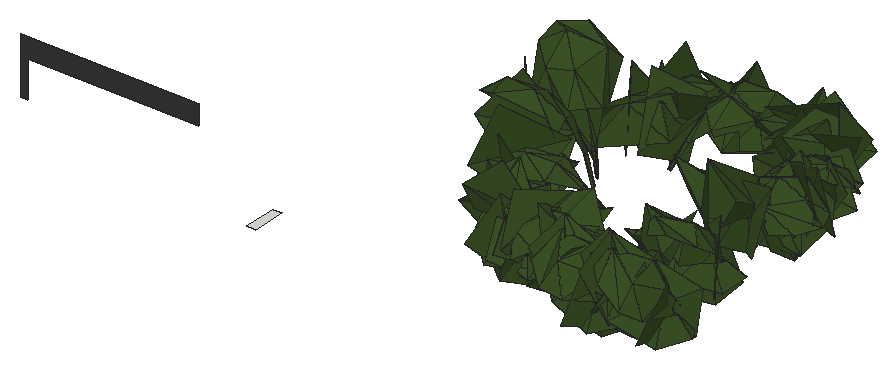
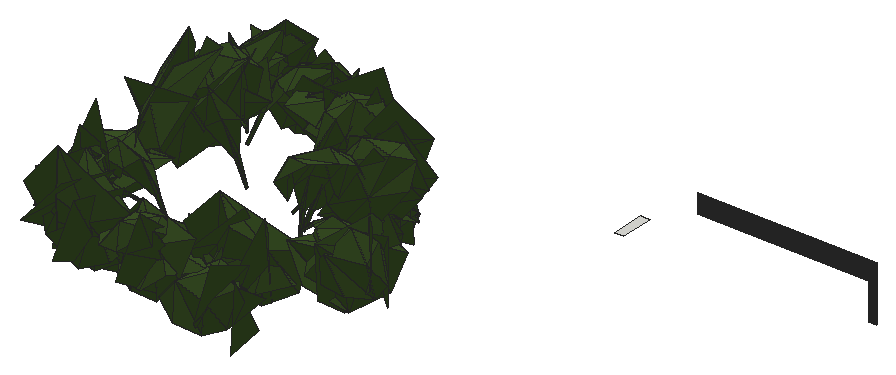
# SketchUp Ruby script. Lengths in inches.
U = 1.inch
M = Sketchup.active_model
def pt(a) = Geom::Point3d.new(a.map { |v| v * U })
def face(e, loops, mat)
  f = e.add_face(loops[0].map { |a| pt(a) })
  loops[1..].each { |l| e.add_face(l.map { |a| pt(a) }).erase! }
  f.material = f.back_material = mat if mat
  f
end
# faces: each face lists its corners as indices into pts; further lists are holes
def faces(e, pts, list, mat = nil) = list.each { |f| face(e, (f[0].is_a?(Array) ? f : [f]).map { |l| l.map { |i| pts[i] } }, mat) }
# xy, xz, yz: faces in a plane at the given z, y or x. An outline is a flat list of corners, or four numbers for a rectangle; further outlines are holes
def ring(l) = l.size == 4 ? [[l[0], l[1]], [l[2], l[1]], [l[2], l[3]], [l[0], l[3]]] : l.each_slice(2).to_a
def flat(e, list, mat, &to3) = list.each { |f| face(e, (f[0].is_a?(Array) ? f : [f]).map { |l| ring(l).map { |u, v| to3.(u, v) } }, mat) }
def xy(e, z, list, mat = nil) = flat(e, list, mat) { |x, y| [x, y, z] }
def xz(e, y, list, mat = nil) = flat(e, list, mat) { |x, z| [x, y, z] }
def yz(e, x, list, mat = nil) = flat(e, list, mat) { |y, z| [x, y, z] }
def lines(e, pts, list) = list.each { |a, b| e.add_line(pt(pts[a]), pt(pts[b])) }
# prism: a flat outline (further loops are holes) pulled along v
def prism(e, loops, v, mat = nil)
  f = face(e, loops, mat); d = Geom::Vector3d.new(v.map { |x| x * U })
  f.pushpull(f.normal.samedirection?(d) ? d.length : -d.length)
end
def box(e, o, s, mat = nil) = prism(e, [[o, [o[0] + s[0], o[1], o[2]], [o[0] + s[0], o[1] + s[1], o[2]], [o[0], o[1] + s[1], o[2]]]], [0, 0, s[2]], mat)
def at(x, y, z, deg = 0) = Geom::Transformation.translation(pt([x, y, z])) * Geom::Transformation.rotation(ORIGIN, Z_AXIS, deg.degrees)
def axes(o, x, y, z) = Geom::Transformation.new([*x, 0, *y, 0, *z, 0, *pt(o).to_a, 1])
def part(name) = M.definitions.add(name)
# library, detail: a bought-in or finely detailed component or shape, given as its bounding box
def library(name, o, s) = part(name).tap { |d| box(d.entities, o, s) }
def detail(e, o, s) = box(e.add_group.entities, o, s)
def put(e, d, t, mat = nil) = e.add_instance(d, t).tap { |i| i.material = mat if mat }
def group(e, t, mat = nil) = e.add_group.tap { |g| g.transformation = t; g.material = mat if mat }.entities
root = M.entities
M.materials.add("AM113_062_Tilia").color = [58, 81, 37]
M.materials.add("[Color M07]").color = [58, 58, 58]
xy(root,573.56,[[1069.1,76.875,1085.03,135.5625]])
xz(root,139.5,[[622.42,592.47,635.92,592.47,635.92,656.55,935.92,656.55,935.92,690.29,622.42,690.29]],"[Color M07]")
p = [[1443.51,292.98,646.41],[1464.43,234.21,547.76],[1450.95,156.04,585.71],[1313.8,681.43,653.64],[1309.07,696.98,547.83],[1320.91,620.27,548.11],
  [1397.61,604.9375,611.74],[1427.87,323.96,609.64],[1351.07,283.39,549.18],[1310.29,240.17,626.87],[1598.13,326.94,592.23],[1582.61,322.04,549.59],
  [1579.03,323.87,550.71],[1677.45,585.75,568.42],[1629,613.75,550.49],[1636.24,630.1,611.62],[1596.64,636.71,572.14],[1594.52,326.77,598.71],
  [1580.72,319.99,550.67],[1595.26,320.34,602.37],[1258.51,510.73,551.17],[1251.36,439.39,561.68],[1236.11,459.66,636.62],[1233.45,517.74,632.64],
  [1272.77,558.58,675.32],[1248.99,581.45,603.9],[1305.23,287.85,592.1875],[1320.3125,291.58,551.625],[1415.08,289.36,555.38],[1407.94,207.2,551.82],
  [1455.12,191.39,578.6],[1415.6875,218.73,631.61],[1349.93,247.89,569.4375],[1311.66,302.61,664.74],[1286.19,323.64,565.63],[1362.78,317.03,551.82],
  [1403.5625,372.15,631.88],[1407.33,211.96,682.55],[1360.55,192.08,596.88],[1425.15,218.16,552.73],[1441.07,302.9,595.82],[1334.58,363.64,552.66],
  [1349.65,351.35,575.07],[1245.76,399.61,631.15],[1253.6875,405.07,587.64],[1648.32,148.625,588.42],[1701.22,189.58,553.52],[1717.44,188,632.54],
  [1741.49,222.52,571.75],[1318.54,309.23,554.29],[1351.14,271.29,577.23],[1344.81,319.46,627.41],[1292.03,376.14,578.625],[1551.52,167.6875,572.65],
  [1622.27,164.6875,554.71],[1622.07,156.6,635.81],[1670.73,165.67,585.16],[1608.22,634.78,584.17],[1593.65,627.43,554.78],[1518.56,630.32,567.47],
  [1689.5,596.59,578.69],[1643.92,630.1875,555.32],[1632.76,621.09,617.87],[1607.43,646.57,573.52],[1427.62,288.11,584.83],[1398.75,394.55,650.45],
  [1332.55,410.9,558.42],[1259.05,385.79,601.68],[1671.8,430.75,670.73],[1715.42,419.11,611.41],[1701.56,489.56,559.68],[1708.06,482.24,646.89],
  [1690.78,537.73,651.45],[1688.71,559.6,574.74],[1650.81,649.24,640.19],[1616.11,607.86,560.91],[1612.67,563.04,636.5625],[1672.51,633.65,561.2],
  [1734.08,169.8,674.68],[1707.04,133.81,583.77],[1699.45,209.03,561.15],[1647.57,247.13,646.8],[1245.64,400.8,609.69],[1241.04,522.07,562.47],
  [1225.44,449.43,567.67],[1248.78,462.16,641.78],[1261,517.78,645.96],[1329.3125,547.83,657.625],[1273.2,583.09,620.53],[1617.14,133.8,679.1875],
  [1587.32,119.06,580.21],[1632.02,181.21,563.7],[1604.22,247.01,639.46],[1210.07,475.86,671.57],[1206.76,480.65,563.96],[1266.11,431.64,576.89],
  [1656.21,132.66,606.36],[1714.59,166.9,566.49],[1708.17,196.93,637.89],[1748.77,206.47,578.3],[1582.25,254.84,657.16],[1535.71,202.89,567.07],
  [1519.56,128.38,614.375],[1510.49,634.69,591.6],[1228.92,408.3125,610.75],[1544.88,151.1,590.5],[1616.28,139.24,568.27],[1619.89,169.58,639.79],
  [1665.22,148.92,591.68],[1685.63,580.37,679.45],[1721.08,579.5625,631.29],[1677.88,614.08,628.61],[1367.26,245.6875,654.63],[1365.33,306.9,685.07],
  [1311.15,286.05,649],[1436.14,578.91,615.29],[1419.1,564.17,572.02],[1422.32,566.01,569.39],[1443.08,579.84,613.99],[1411.87,507.45,616.69],
  [1427,597.97,569.84],[1419.51,648.93,656.41],[1401.61,217.16,660.34],[1407.96,178.55,594.29],[1483.48,205.09,569.99],[1460.63,189.48,650.56],
  [1510.52,212.32,675.7],[1545.93,224.17,609.62],[1433.23,582.59,610.09],[1420.1,567.83,569.98],[1702.87,325.8,701.78],[1734.15,271.99,629.74],
  [1694.96,320.6,570.26],[1608.11,323.67,611.05],[1404.69,590.07,602.44],[1420,567.67,570.29],[1422.37,565.58,573.67],[1408.09,591.89,608.67],
  [1422.63,568.91,570.32],[1410.42,598.4,606.78],[1537.44,604.97,675.28],[1572.25,640.36,622.27],[1506.85,669.99,570.53],[1513.58,664.625,657.96],
  [1457.21,678.96,661.32],[1440.11,694.91,585.32],[1734.57,245.75,634.83],[1589.54,628.5625,626.63],[1566.26,151.12,656],[1534.45,192.81,706.91],
  [1497.74,160.84,652.42],[1337.85,585.41,704.22],[1329.92,580.04,572.72],[1386.99,511.43,603.95],[1350.2,642.21,626.66],[1625.55,551.38,653.18],
  [1674.04,555.13,573.11],[1717.16,604.83,593.07],[1577.36,604.36,599.32],[1682.61,244.96,607.61],[1709.5,306.51,573.58],[1695.23,324.09,649.96],
  [1713.875,359.28,586.7],[1420.15,231.41,629.71],[1443.73,181.66,592.26],[1480.47,238.94,573.85],[1386.78,344.77,633.36],[1643.25,658.28,592.23],
  [1572.71,665.11,574.65],[1574.02,676.53,655.0625],[1524.52,668.54,605.5],[1673.92,594.75,623.91],[1332.02,600.27,574.98],[1290.67,570.71,598.18],
  [1337.29,579.57,651.97],[1400.17,618.76,594.16],[1307.52,379.79,665.22],[1339.48,739.58,605.03],[1351.89,716.07,575.52],[1345.45,626.48,614.82],
  [1393.23,192.09,575.94],[1339.23,241.38,593.7],[1681.91,325.2,647.35],[1661.93,372.01,576.92],[1578.9,268.6,663.63],[1725.6875,352.8,602.75],
  [1326.74,473.71,648.78],[1620.84,430,631.93],[1689.64,410.93,617.64],[1717.91,481.57,576.97],[1679.54,475.125,648.7],[1678.47,532.12,651.28],
  [1713.77,555.13,590.34],[1569.31,506.47,577.08],[1595.71,496.77,618.41],[1591.39,502.18,620.2],[1566.29,508.27,580.12],[1412.41,301.56,593.78],
  [1592.51,506.53,614.71],[1569.72,509.33,577.55],[1710.96,263.47,594.42],[1475.375,225.97,626.38],[1326.26,369.39,653.71],[1368.29,430.22,671.25],
  [1297.03,432.2,656.2],[1661.52,540.46,669.35],[1711.1875,564.33,647.2],[1666.25,596.42,641.89],[1401.1875,271.04,628.78],[1395.31,202.45,600.54],
  [1474.8,186.42,581.99],[1449.46,216.625,653.24],[1503.45,223.83,675.08],[1542.17,197.47,620.16],[1710.89,525.17,694.47],[1669.76,562.73,583.64],
  [1607.46,503.16,626.85],[1739.39,529.24,593.19],[1569.95,629.45,636.38],[1358.07,303.1,648.12],[1580.74,700.72,696.75],[1561.98,649.66,584.85],
  [1586.03,585.43,664.88],[1610.71,709.37,596.67],[1670.9,190.7,647.71],[1344.42,568.48,648.13],[1290.3125,584.26,614.1],[1312.11,522.16,585.18],
  [1454.02,524.4,642.36],[1400.84,697.04,632.89],[1460.75,187.87,691.92],[1580.43,690.65,586.38],[1531.14,685.15,610.8],[1575.4,663.61,659.93],
  [1651.07,675.11,608.85],[1674.85,378.48,629.22],[1331.39,732.74,586.95],[1311.16,703.53,590],[1343.63,712.8,627.5],[1401.89,703.51,635.34],
  [1374.5625,741.53,596.15],[1638.27,165.375,725.99],[1623.05,114.34,679.17],[1681.48,149.97,665.45],[1590.34,308.6,628.8],[1648.1,234.86,588.7],
  [1698.09,218.15,674.0625],[1607.59,576.93,682.92],[1656.71,621.94,589],[1677.98,697.1,630.91],[1628.48,240.48,670.01],[1613.44,165.6875,589.25],
  [1654.67,100.59,634.3],[1323.23,658.78,631.6875],[1310.75,617.35,601.5],[1355.5,616.09,589.78],[1361.42,617.57,626.85],[1521.66,678.17,589.86],
  [1504.56,636.68,655.53],[1512.56,564.72,629.45],[1565.43,613.81,624.6],[1455.51,665.64,659.27],[1456.5625,712.43,604.28],[1418.87,377.28,621.66],
  [1441.56,393.11,590.28],[1444.49,394.15,593.74],[1690.97,591.08,631.26],[1535.81,247.38,677.46],[1498.15,186.48,665.15],[1567.13,179.79,664.46],
  [1441.07,395.85,591.375],[1412.8,383.66,629.42],[1418.58,379.6,629.05],[1477.03,685.85,706.65],[1427.18,679.86,591.54],[1443.55,592.45,624.2],
  [1491.9375,720.14,610.16],[1670.01,217.59,604.37],[1195.53,534.55,616.75],[1223.15,524.39,592.14],[1273.59,454.92,644.13],[1618.72,328.89,647.23],
  [1642.03,337.64,631.88],[1630.22,679.2,674.42],[1659.65,637.71,727.91],[1697.93,664.93,671],[1384.81,395.16,681.5],[1343.9,337.13,593.07],
  [1277.85,301.75,643.74],[1669.04,629.77,652.16],[1673.65,642.61,593.6],[1606.52,625.8125,596.25],[1637.53,632.69,626.12],[1683.17,629.46,634.47],
  [1700.18,634.11,601.1],[1382.07,270.86,649.95],[1324.8,309.88,649.67],[1376.87,449.35,640.75],[1380.84,454.38,593.95],[1384.8,453.3125,593.68],
  [1381.67,450.58,645.53],[1382.44,456.8,594.1875],[1380.53,456.97,649.13],[1388.8,598.52,677.04],[1438.35,559.49,700.41],[1455.2,617.95,672.99],
  [1600.88,206.8,700.62],[1394.6875,428.1875,594.375],[1371.38,436.66,639.11],[1378.33,436.24,640.72],[1398.3,429.89,596.16],[1607.68,262.43,628.41],
  [1605.93,288.89,595.42],[1606.47,292.07,598.71],[1380.12,430.57,638.53],[1396.36,426.28,596.23],[1426.99,707.44,602.67],[1615.34,591.02,604.8],
  [1603.31,289.9,596.41],[1599.01,260.71,636.1],[1605.45,263.61,635.7],[1409.32,632.33,626.29],[1419.72,648.83,598.1],[1305.8125,529.12,639.36],
  [1284.2,318.38,608.12],[1367.5625,295.82,599.25],[1333.92,310.78,641.32],[1379.69,339.84,600.98],[1195.83,523.45,599.19],[1199.82,488.34,604.93],
  [1214.04,518.21,643.44],[1262.56,550.53,657.56],[1221.1,559.15,610.64],[1705.125,633.71,618.03],[1692.52,613.23,599.47],[1618.82,605.9,620.11],
  [1352.55,450.73,646.08],[1292.89,380.51,600.45],[1233.77,371.24,677.59],[1690.96,240.12,633.97],[1727.13,299.76,600.57],[1383.13,338.05,638.53],
  [1654.2,325.58,601.12],[1690.44,328.08,666.88],[1692.1875,349.98,610.1],[1686.46,587.33,662.16],[1714.25,607.17,625.16],[1304.98,336.21,676.01],
  [1329.63,618.73,602.28],[1402.04,628.8,620.17],[1604.96,305.33,644.4],[1386.43,622.24,640.63],[1717.08,135.97,624.78],[1724.5,220.66,603.1875],
  [1719.94,188.625,650.98],[1679.71,226.09,612.375],[1674.67,332.87,637.79],[1672.13,399.99,603.76],[1693.54,410.98,679.41],[1674.55,451.89,622.35],
  [1412.68,708.89,642.54],[1613.85,595.01,634.57],[1255.23,424.49,629.37],[1234.17,464.61,654.05],[1336.97,621.25,645.91],[1339.13,702.98,682.05],
  [1523.19,646.21,669.71],[1638.95,260.6,636.21],[1616.4,278.07,606.14],[1615.27,281.06,609.46],[1609,135.24,693.36],[1665.28,173.24,675.55],
  [1619.76,264.94,718.63],[1652.84,212.23,697.04],[1679.46,275.62,686.26],[1613.91,277.27,607.8125],[1634.55,254.29,645.72],[1637.53,260.55,643.98],
  [1477.8,335.71,607.9375],[1464.27,304.61,641.27],[1468.5,309.3125,645.34],[1478.52,338.59,611.82],[1287.31,343.15,655.73],[1261.38,344.66,617.88],
  [1416.5625,208.28,650.69],[1403.6875,215.93,608.64],[1433.32,161.18,618.68],[1436.86,264.24,619.17],[1627.5625,651.04,684.87],[1654.55,582.2,702.32],
  [1695.97,639.93,685.5],[1258.59,350.07,639.14],[1281.81,362.375,609.17],[1369.27,327.64,624.35],[1473.88,309.22,641.39],[1480.51,335.57,609.3],
  [1568.1,237.98,670.46],[1385.53,239.5,687.73],[1264.81,414.83,673.07],[1726.25,284.39,668.44],[1453.86,602.36,658.85],[1439.55,625.52,652.96],
  [1281.77,569.13,626.72],[1295.37,403.99,636.57],[1522.03,617.56,628.29],[1694.07,328.74,651.77],[1699.44,395.875,611],[1681.61,409.43,687.38],
  [1692.18,447.31,625.15],[1621.68,156.3,654.53],[1652.14,176.24,611.875],[1620.34,209.02,611.06],[1623.16,212.39,648.52],[1493.04,186.94,710.4375],
  [1520.39,169.03,611.16],[1544.5625,242.36,621.45],[1590.32,116.16,622.97],[1603.61,552.625,631.45],[1592.68,529.76,612.12],[1591.2,528.31,615.4],
  [1750.8,475.49,646.1875],[1728.34,481.07,612.1875],[1653.23,533.49,643.97],[1684.9375,232.69,648.67],[1633.23,461.48,612.39],[1676.95,422.125,620.59],
  [1683.34,442.13,658.1],[1621.82,476.91,640.93],[1534.26,621.72,664.64],[1472.93,589.58,639.63],[1492.99,593.34,612.53],[1549.15,608.78,625.99],
  [1605.02,551.93,637.49],[1594.14,528.17,613.25],[1610.64,551.34,637.42],[1584.66,145.4375,689.13],[1460.29,146.66,642.59],[1469.02,172.69,614.44],
  [1502.62,249.57,671.49],[1435.49,248.5625,614.375],[1452.15,244.96,639.84],[1334.5,220.17,670.29],[1342.65,233.23,629.64],[1624.22,500.125,659.39],
  [1635.7,524.41,651.24],[1723.19,412.03,715.78],[1722.14,368.95,623.33],[1657.16,410.89,614.84],[1606.54,394.27,712.33],[1342.71,467.09,642.42],
  [1372.01,459.6,615.26],[1374.81,459.76,619.13],[1343.42,470.93,648.61],[1373.13,462.29,615.33],[1341.03,477.25,645.94],[1642.31,533.22,616.12],
  [1689.83,532.0625,668.65],[1666.27,568.18,638.11],[1373.04,584.96,708.59],[1267.6875,446.43,675.01],[1211.8,509.76,698.59],[1312.47,393.92,678.32],
  [1265.33,385.18,641.46],[1610.04,617.38,639.46],[1669.27,642.05,672.39],[1475.11,148.58,630.68],[1444.57,274.48,653.15],[1436.71,638.55,619.2],
  [1460.95,673.79,678.15],[1418.9,675.43,645.29],[1565.5625,220.06,674.29],[1399.26,571.96,667.86],[1465.41,592.59,669.4],[1734.38,446.41,629.51],
  [1470.42,292.94,650.17],[1386.56,359.68,660.19],[1290.36,453.09,621.75],[1290.11,459.39,658.76],[1660.53,460.8,689.41],[1555.98,110.14,632.39],
  [1569.97,133.02,669.25],[1645.22,572.19,676.24],[1374.75,312.07,650.4],[1696.2,110.35,641.89],[1697.51,139.04,676.27],[1627.1,454.04,655.54],
  [1697.6,563.32,647.98],[1558.4375,669.31,643.6],[1644.53,608.98,653.51],[1361.87,660.45,648.4],[1315.51,520.61,630.47],[1605.99,227.04,669],
  [1680.85,299.71,713.57],[1544.35,286.25,676.7],[1381.76,386.39,655.54],[1751.82,487.5,629.7],[1387.27,644.78,631.03],[1723.7,485.28,664.8],
  [1738.41,520.27,634.69],[1622.56,578.66,629.78],[1315.9,502.36,660.03],[1462.3,172.68,666.96],[1503.68,165,648.11],[1612.46,687.43,707.24],
  [1620.83,581.1,654.74],[1653.27,316.51,682.59],[1538.69,181.18,688.43],[1522.77,134.87,653.89],[1403.15,656.75,680.27],[1626.54,220,694.875],
  [1651.69,283.33,678.6],[1703.58,159.06,693.1],[1607.5,277.02,635.22],[1621.95,234.52,684.95],[1636.28,262.57,707.09],[1366.27,405.75,635.42],
  [1312.53,425.08,655.38],[1580.6,236.26,663.29],[1665.58,234.51,673.94],[1634.39,563.96,653.65],[1673.11,334.73,777.62],[1696.53,290.96,724.6],
  [1704.21,358.83,709.85],[1651.86,554.27,637.93],[1319.67,436.62,638.32],[1261.54,441.55,651.11],[1272.79,440.125,695.01],[1340.24,444.35,663.31],
  [1344.12,343.87,669.12],[1355.39,435.33,690.32],[1363,409.87,699.93],[1300.31,325.4,704.35],[1478.13,636.91,681.79],[1391.625,235.75,718.53],
  [1370.35,447.06,701.23],[1346.8125,433.27,695.86],[1668.08,498.0625,676.24],[1463.61,272.96,678.44],[1490.07,265.14,677.46],[1646.23,157.92,706.03],
  [1658.52,109.98,672.73],[1304.18,480.06,673.83],[1502.9375,250.81,705.09],[1454.66,180.27,721.52],[1556.31,232.01,642.9],[1512.16,196.19,664.05],
  [1260.02,492.25,673.64],[1532.71,705.67,647.23],[1317.42,319.52,743.71],[1649.69,540.74,675.96],[1497.66,711.26,651.05],[1639.78,225.41,675.125],
  [1506.1875,262.99,645.91],[1501.65,210.96,690.43],[1538.83,241.18,676.04],[1290.37,407.23,752.69],[1711.31,489.88,718.45],[1518.64,677.98,678.06],
  [1597.99,182.79,680.34],[1688.94,195.86,683.88],[1377.92,472.49,692.56],[1464.55,227.86,688.79],[1236.68,397.69,699.27],[1614.9,332.21,764.36],
  [1673.61,293.22,743.93],[1677.6,360.97,725.83],[1532.4,258.72,716.49],[1621.25,205.68,660.69],[1613.33,151.49,689.58],[1323.02,419.34,726.69],
  [1693.23,279.13,706.44],[1719.72,253.41,689.48],[1307.47,435.93,747.71],[1297.4,410.67,694.83],[1326.1,440.97,670.9],[1329.77,382.12,746.37],
  [1369.59,359.1875,723.74],[1361.99,386.31,677.35],[1354.23,512.51,763.31],[1367.87,499.2,684.02],[1357.1,541.26,735.88],[1682.68,231.59,704.92],
  [1343.5,455.04,747.99],[1265.63,472.29,761.87],[1251.87,361.36,726.37],[1273.04,392.45,740.53],[1284.21,349.37,737.81],[1304.16,534.25,778.36],
  [1304.05,485.82,785.19],[1270.34,505.14,778.57]]
faces(root,p,[[0,1,2],[3,4,5],[3,5,6],[7,8,9],[10,11,12],[13,14,15],[14,16,15],[17,12,18],
  [18,19,17],[12,17,10],[20,21,22],[22,23,20],[20,23,24],[24,25,20],[26,27,28],[29,30,31],
  [32,29,31],[33,34,35],[33,35,36],[37,38,39],[37,39,40],[41,42,43],[43,44,41],[45,46,47],
  [46,48,47],[49,50,51],[52,49,51],[53,54,55],[54,56,55],[57,58,59],[60,61,62],[61,63,62],
  [28,64,26],[65,66,67],[68,69,70],[70,71,68],[72,71,70],[70,73,72],[74,75,76],[74,77,75],
  [78,79,80],[78,80,81],[21,82,22],[83,84,85],[85,86,83],[83,86,87],[87,88,83],[89,90,91],
  [89,91,92],[93,94,95],[96,97,98],[97,99,98],[100,101,102],[59,103,57],[84,104,85],[105,106,107],
  [106,108,107],[109,110,13],[13,111,109],[15,111,13],[31,112,32],[32,112,113],[113,114,32],[115,116,117],
  [117,118,115],[119,120,121],[122,123,124],[124,125,122],[126,125,124],[124,127,126],[128,129,116],[130,131,132],
  [130,132,133],[134,135,136],[137,136,138],[138,139,137],[140,141,142],[142,143,140],[144,143,142],[142,145,144],
  [47,48,146],[116,115,128],[15,16,147],[53,148,149],[55,148,53],[149,150,53],[151,152,153],[151,154,152],
  [155,156,157],[62,63,158],[159,160,161],[160,162,161],[136,137,134],[163,164,165],[163,165,166],[167,168,169],
  [168,170,169],[73,171,72],[172,173,174],[175,172,174],[42,176,43],[177,178,179],[180,164,163],[181,180,163],
  [182,183,184],[182,185,183],[93,95,186],[187,188,189],[189,190,187],[191,190,189],[189,192,191],[193,194,195],
  [195,196,193],[51,50,197],[198,199,196],[98,99,200],[31,30,201],[51,202,52],[52,202,203],[203,204,52],
  [205,206,60],[60,207,205],[62,207,60],[196,195,198],[208,209,210],[210,211,208],[212,211,210],[210,213,212],
  [214,215,216],[214,217,215],[103,218,57],[64,219,26],[220,221,222],[220,223,221],[55,56,224],[225,226,227],
  [225,227,228],[145,229,144],[230,0,2],[231,232,233],[234,231,233],[161,162,235],[236,237,238],[239,240,236],
  [236,238,239],[241,242,45],[45,243,241],[47,243,45],[244,245,246],[247,248,249],[250,251,252],[253,254,255],
  [255,256,253],[257,258,259],[259,260,257],[261,258,257],[257,262,261],[237,254,253],[238,237,253],[263,264,265],
  [192,266,191],[267,268,105],[105,269,267],[107,269,105],[270,271,272],[272,265,270],[273,274,275],[273,276,274],
  [107,108,277],[278,279,280],[10,17,281],[281,282,10],[167,283,284],[284,285,167],[169,283,167],[286,287,288],
  [289,155,157],[290,291,292],[293,290,292],[294,290,293],[163,295,181],[166,296,181],[181,295,166],[265,272,263],
  [297,298,299],[299,300,297],[300,299,301],[51,197,203],[301,302,300],[175,303,304],[304,305,175],[174,303,175],
  [98,200,306],[307,308,309],[309,310,307],[311,312,313],[314,315,310],[310,309,314],[239,316,240],[292,291,317],
  [318,319,320],[320,313,318],[239,321,322],[322,316,239],[174,173,323],[313,320,311],[281,17,19],[324,325,326],
  [326,325,327],[328,329,330],[328,330,331],[331,332,328],[62,158,205],[333,334,335],[336,337,338],[339,340,182],
  [340,185,182],[327,341,326],[342,282,343],[343,344,342],[294,293,345],[345,346,294],[347,65,67],[348,226,225],
  [349,348,225],[19,350,281],[351,256,134],[134,137,351],[352,353,354],[354,353,355],[356,357,358],[357,359,358],
  [262,360,261],[107,277,267],[317,361,292],[329,362,363],[330,329,363],[179,364,177],[364,365,177],[169,170,366],
  [367,368,369],[306,370,96],[96,371,306],[98,371,96],[351,137,139],[139,321,351],[372,373,159],[159,374,372],
  [161,374,159],[375,376,377],[377,369,375],[378,379,380],[380,381,378],[382,324,326],[383,324,382],[384,385,386],
  [387,385,384],[234,388,389],[389,390,234],[233,388,234],[391,392,393],[394,395,381],[369,377,367],[127,396,126],
  [397,7,9],[22,82,398],[399,344,343],[128,115,400],[400,401,128],[331,402,332],[85,104,403],[233,232,404],
  [405,406,407],[406,408,407],[409,410,411],[411,412,409],[413,414,415],[15,147,109],[109,111,15],[381,380,394],
  [416,410,409],[417,418,419],[420,421,422],[355,423,354],[424,425,426],[426,427,424],[428,429,430],[430,431,428],
  [432,419,433],[433,434,432],[400,115,118],[118,429,400],[435,100,102],[436,437,438],[439,440,441],[441,442,439],
  [198,195,443],[443,444,198],[445,446,447],[445,447,448],[449,450,451],[452,451,453],[453,454,452],[419,432,417],
  [455,444,456],[456,457,455],[458,119,121],[280,459,278],[459,460,278],[383,382,461],[461,462,383],[205,207,62],
  [335,463,333],[463,464,333],[194,427,443],[443,195,194],[384,386,465],[451,452,449],[384,466,387],[467,401,468],
  [468,469,467],[213,470,212],[349,471,228],[228,472,349],[225,471,349],[426,425,473],[413,415,474],[475,341,263],
  [263,272,475],[363,362,476],[476,477,363],[358,359,478],[479,416,480],[480,416,409],[72,171,481],[393,482,391],
  [483,352,484],[484,352,354],[407,408,485],[345,486,346],[428,431,487],[488,292,361],[488,293,292],[489,351,321],
  [321,239,489],[31,201,113],[490,402,331],[489,253,256],[489,256,351],[203,202,51],[489,238,253],[239,238,489],
  [233,404,389],[491,412,311],[311,320,491],[208,211,212],[492,244,246],[212,493,208],[475,272,271],[161,235,372],
  [271,494,475],[426,473,495],[261,496,259],[259,258,261],[166,295,163],[495,497,426],[495,498,497],[191,499,187],
  [191,266,499],[331,500,490],[465,501,384],[465,502,501],[503,247,249],[261,360,496],[417,432,504],[504,361,417],
  [113,112,31],[505,282,281],[505,343,282],[187,190,191],[506,507,479],[479,480,506],[241,243,47],[47,146,241],
  [24,23,22],[144,229,508],[184,509,339],[339,510,184],[182,510,339],[511,250,252],[345,293,488],[488,361,504],
  [497,498,456],[498,457,456],[512,513,514],[514,350,512],[461,494,515],[515,516,461],[491,320,319],[149,148,55],
  [55,224,149],[319,517,491],[518,423,367],[367,377,518],[85,403,87],[22,398,24],[504,432,434],[434,519,504],
  [520,521,356],[356,522,520],[358,522,356],[306,371,98],[345,519,523],[523,486,345],[524,525,526],[526,527,524],
  [528,326,341],[528,341,475],[529,530,314],[314,309,529],[482,531,391],[308,527,529],[529,309,308],[174,323,304],
  [532,400,429],[429,428,532],[267,269,107],[440,533,441],[534,535,297],[297,300,534],[427,426,536],[536,443,427],
  [379,466,537],[537,380,379],[528,382,326],[537,538,394],[394,380,537],[461,516,462],[87,86,85],[539,540,483],
  [483,484,539],[541,477,449],[449,452,541],[228,471,225],[542,543,436],[438,542,436],[544,545,506],[506,517,544],
  [546,330,363],[331,330,546],[428,487,547],[548,286,288],[518,377,376],[422,549,420],[350,514,505],[505,281,350],
  [550,469,468],[534,300,302],[376,551,518],[552,538,553],[553,554,552],[541,452,454],[454,500,541],[555,336,338],
  [549,556,420],[68,71,72],[547,557,428],[547,550,557],[184,510,182],[501,502,553],[502,554,553],[558,409,412],
  [558,412,491],[559,354,423],[559,423,518],[302,560,534],[372,374,161],[122,125,126],[384,501,561],[466,384,561],
  [559,484,354],[557,550,468],[526,525,562],[536,444,443],[536,456,444],[72,481,68],[563,564,405],[405,565,563],
  [407,565,405],[304,303,174],[532,401,400],[532,468,401],[561,537,466],[488,504,519],[519,345,488],[506,545,507],
  [546,363,477],[558,480,409],[169,366,284],[284,283,169],[407,485,563],[494,461,528],[528,475,494],[461,382,528],
  [500,331,546],[140,143,144],[426,497,536],[546,477,541],[389,388,233],[546,541,500],[126,566,122],[567,568,539],
  [539,551,567],[144,508,140],[517,506,558],[558,491,517],[527,526,569],[569,529,527],[428,557,532],[536,497,456],
  [505,570,343],[570,399,343],[561,501,553],[571,399,570],[506,480,558],[126,396,566],[572,573,574],[574,535,572],
  [539,568,540],[559,518,551],[212,470,493],[551,539,559],[539,484,559],[575,576,577],[577,530,575],[561,553,538],
  [561,538,537],[532,557,468],[358,478,520],[520,522,358],[514,570,505],[578,560,579],[579,580,578],[514,513,581],
  [563,565,407],[514,581,571],[571,570,514],[569,530,529],[582,534,560],[560,578,582],[583,573,572],[526,562,584],
  [584,585,526],[526,585,569],[582,572,535],[582,535,534],[569,575,530],[586,576,575],[584,586,585],[569,585,575],
  [578,580,587],[585,586,575],[588,583,572],[582,588,572],[578,588,582],[589,583,588],[589,588,578],[578,587,589]],"AM113_062_Tilia")
